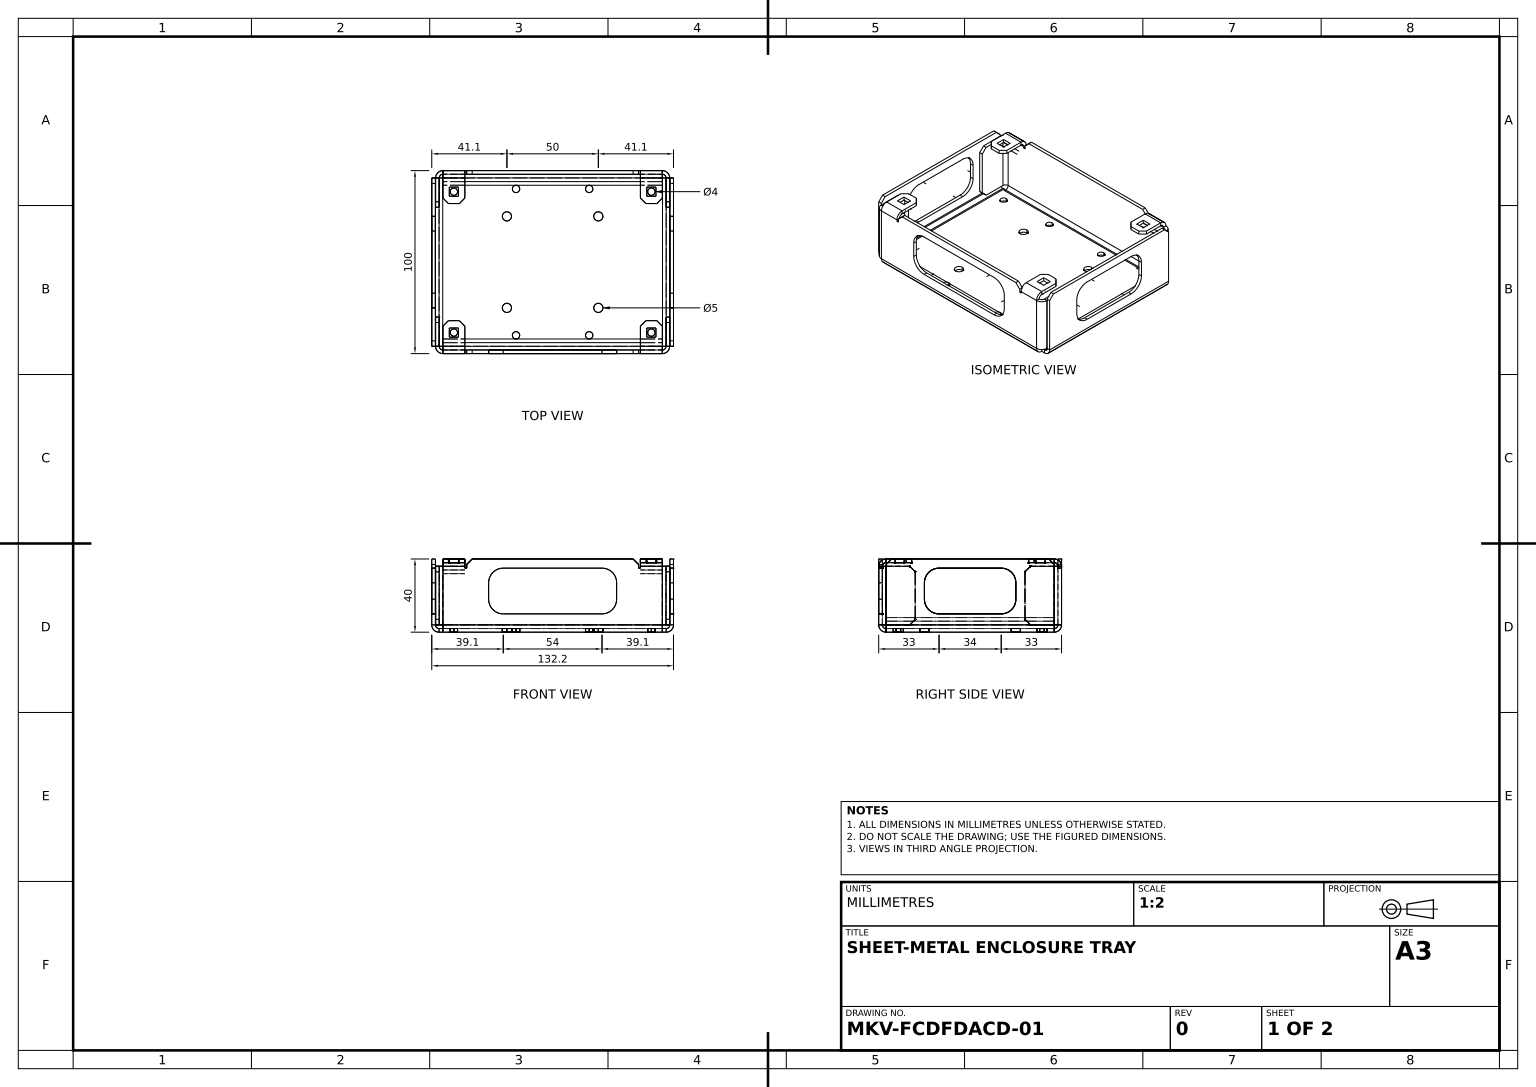
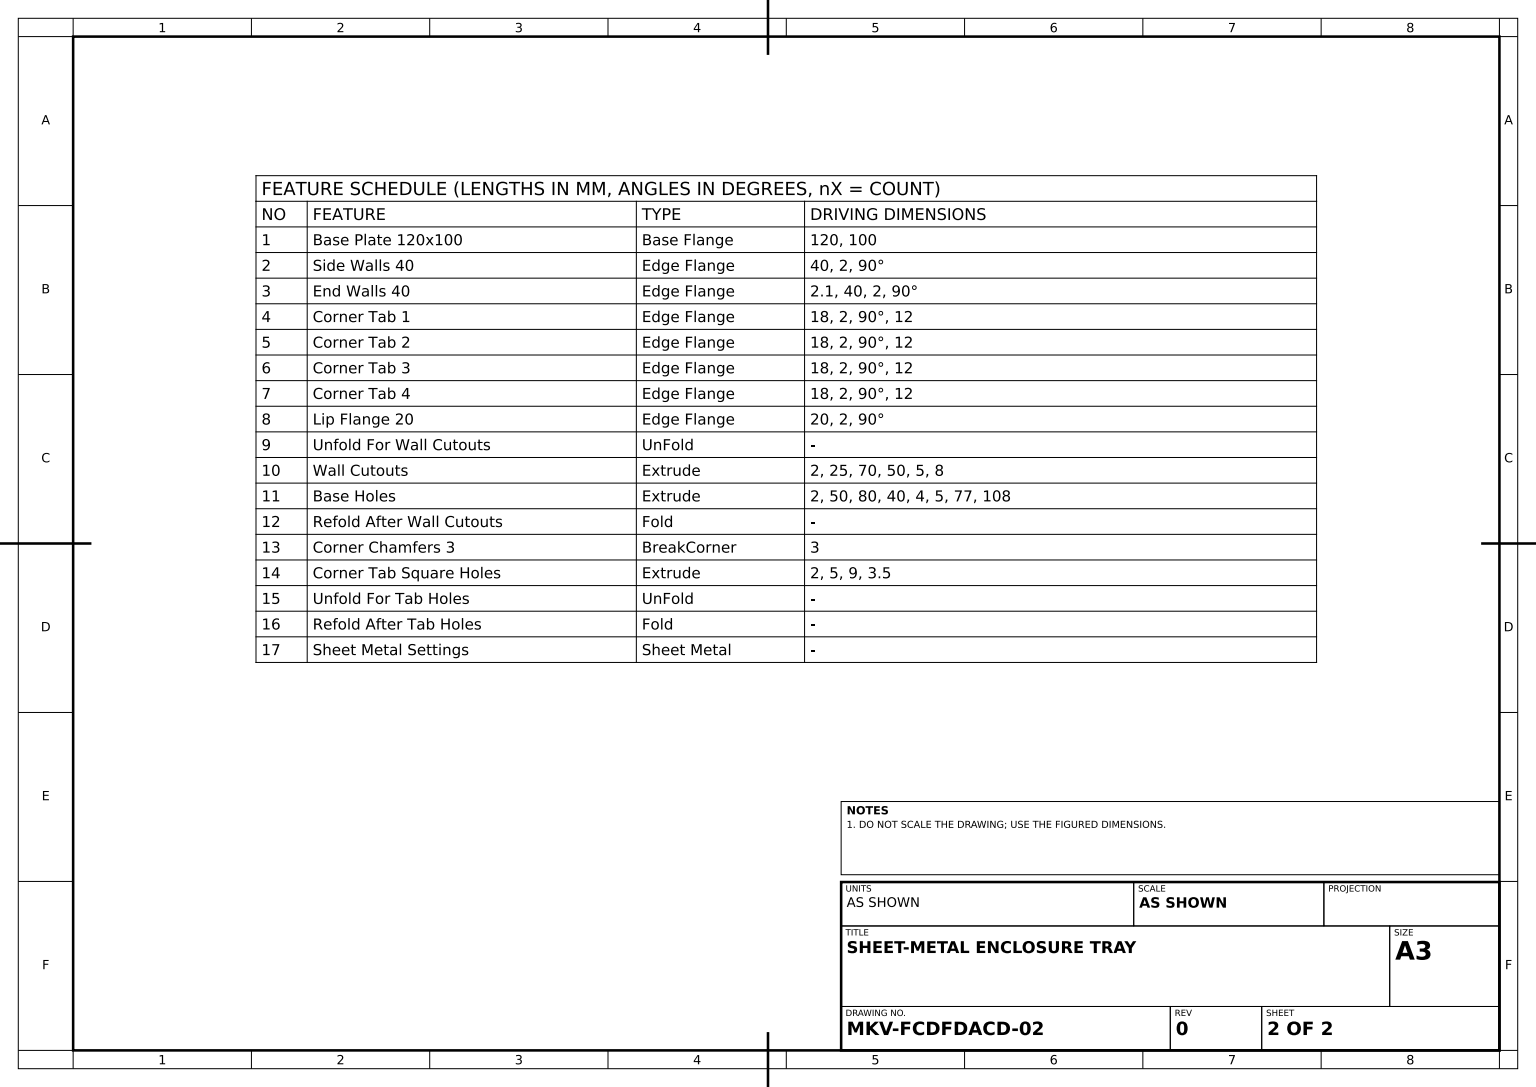
solid
v1 (-48,36,-48)
v2 (-48,38,-46)
e1 v1 v2 CIRCLE(AX(P(-48,36,-46),D(1,0,0),D(0,1,0)),2)
v3 (-48,36,-50)
e2 v1 v3 LINE
v4 (-48,40,-46)
e3 v3 v4 CIRCLE(AX(P(-48,36,-46),D(1,0,0),D(0,-1,0)),4)
e4 v2 v4 LINE
face PLANE(AX(P(-48,36,-46),D(-1,0,0),D(0,-1,0))) rev [-e1 e2 e3 -e4]
v5 (-48,38,46)
v6 (-48,36,48)
e5 v5 v6 CIRCLE(AX(P(-48,36,46),D(1,0,0),D(0,-1,0)),2)
v7 (-48,40,46)
e6 v5 v7 LINE
v8 (-48,36,50)
e7 v7 v8 CIRCLE(AX(P(-48,36,46),D(1,0,0),D(0,0,-1)),4)
e8 v6 v8 LINE
face PLANE(AX(P(-48,36,46),D(-1,0,0),D(0,1,0))) rev [-e5 e6 e7 -e8]
v9 (56.5,38,-41)
v10 (51.5,38,-41)
e9 v9 v10 LINE
v11 (56.5,40,-41)
e10 v9 v11 LINE
v12 (51.5,40,-41)
e11 v11 v12 LINE
e12 v10 v12 LINE
face PLANE(AX(P(56.5,38,-41),D(0,0,-1),D(0,1,0))) rev [-e9 e10 e11 -e12]
v13 (35,27,50)
v14 (35,27,48)
e13 v13 v14 LINE
v15 (35,18,48)
e14 v15 v14 LINE
v16 (35,18,50)
e15 v16 v15 LINE
e16 v16 v13 LINE
face PLANE(AX(P(35,-46.712389,50),D(-1,0,0),D(0,1,0))) [e13 -e14 -e15 e16]
v17 (-62,7,-30)
v18 (-62,4,-33)
e17 v17 v18 LINE
v19 (-64,7,-30)
e18 v19 v17 LINE
v20 (-64,4,-33)
e19 v20 v19 LINE
e20 v18 v20 LINE
face PLANE(AX(P(-64,7,-30),D(0,0.707106781,-0.707106781),D(1,0,0))) rev [-e17 -e18 -e19 -e20]
v21 (48,35,-48)
v22 (48,35,-50)
e21 v21 v22 LINE
v23 (47,35,-50)
e22 v22 v23 LINE
v24 (47,35,-48)
e23 v24 v23 LINE
e24 v24 v21 LINE
face PLANE(AX(P(47,35,-48),D(0,1,0),D(0,0,1))) [e21 e22 -e23 e24]
v25 (66.1,10,17)
v26 (64.1,10,17)
e25 v25 v26 LINE
v27 (64.1,18,25)
e26 v27 v26 CIRCLE(AX(P(64.1,18,17),D(1,0,0),D(0,0,1)),8)
v28 (66.1,18,25)
e27 v28 v27 LINE
e28 v28 v25 CIRCLE(AX(P(66.1,18,17),D(1,0,0),D(0,0,1)),8)
face CYL(AX(P(66.1,18,17),D(-1,0,0),D(0,0,1)),8) rev [e25 -e26 -e27 e28]
v29 (60,0,-46)
v30 (60,4,-50)
e29 v29 v30 CIRCLE(AX(P(60,4,-46),D(1,0,0),D(0,0,1)),4)
v31 (60,4,-48)
e30 v31 v30 LINE
v32 (60,2,-46)
e31 v32 v31 CIRCLE(AX(P(60,4,-46),D(1,0,0),D(0,0,-1)),2)
e32 v32 v29 LINE
face PLANE(AX(P(60,4,-46),D(-1,0,0),D(0,0,1))) rev [e29 -e30 -e31 e32]
v33 (54,0,-40.5)
v34 (54,0,-36.5)
e33 v33 v34 CIRCLE(AX(P(54,0,-38.5),D(0,1,0),D(0,0,1)),2)
v35 (54,2,-40.5)
e34 v33 v35 LINE
v36 (54,2,-36.5)
e35 v35 v36 CIRCLE(AX(P(54,2,-38.5),D(0,1,0),D(0,0,1)),2)
e36 v34 v36 LINE
face CYL(AX(P(54,0,-38.5),D(0,1,0),D(0,0,1)),2) rev [-e33 e34 e35 -e36]
v37 (57,38,-32)
v38 (57,40,-32)
e37 v37 v38 LINE
v39 (60,38,-35)
e38 v39 v37 LINE
v40 (60,40,-35)
e39 v40 v39 LINE
e40 v38 v40 LINE
face PLANE(AX(P(60,40,-35),D(-0.707106781,0,-0.707106781),D(0,-1,0))) rev [-e37 -e38 -e39 -e40]
v41 (51,40,32)
v42 (48,40,35)
e41 v41 v42 LINE
v43 (51,38,32)
e42 v43 v41 LINE
v44 (48,38,35)
e43 v44 v43 LINE
e44 v42 v44 LINE
face PLANE(AX(P(48,40,35),D(0.707106781,0,0.707106781),D(0,-1,0))) rev [-e41 -e42 -e43 -e44]
v45 (-51,38,32)
v46 (-57,38,32)
e45 v45 v46 LINE
v47 (-57,40,32)
e46 v46 v47 LINE
v48 (-51,40,32)
e47 v48 v47 LINE
e48 v48 v45 LINE
face PLANE(AX(P(-60,40,32),D(0,0,1),D(0,-1,0))) rev [e45 e46 -e47 e48]
v49 (64,36,-33)
v50 (64,33,-30)
e49 v49 v50 LINE
v51 (62,36,-33)
e50 v51 v49 LINE
v52 (62,33,-30)
e51 v52 v51 LINE
e52 v50 v52 LINE
face PLANE(AX(P(64,33,-30),D(0,-0.707106781,-0.707106781),D(-1,0,0))) rev [-e49 -e50 -e51 -e52]
v53 (-51,38,-32)
v54 (-51,40,-32)
e53 v53 v54 LINE
v55 (-57,40,-32)
e54 v55 v54 LINE
v56 (-57,38,-32)
e55 v55 v56 LINE
e56 v56 v53 LINE
face PLANE(AX(P(-48,40,-32),D(0,0,-1),D(0,1,0))) rev [e53 -e54 e55 e56]
v57 (-20,2,42)
v58 (-20,2,38)
e57 v57 v58 CIRCLE(AX(P(-20,2,40),D(0,1,0),D(0,0,1)),2)
v59 (-20,0,38)
e58 v59 v58 LINE
v60 (-20,0,42)
e59 v60 v59 CIRCLE(AX(P(-20,0,40),D(0,1,0),D(0,0,1)),2)
e60 v60 v57 LINE
face CYL(AX(P(-20,0,40),D(0,1,0),D(0,0,1)),2) rev [e57 -e58 -e59 e60]
v61 (-62,4,33)
v62 (-62,4,46)
e61 v61 v62 LINE
v63 (-62,7,30)
e62 v61 v63 LINE
v64 (-62,33,30)
e63 v64 v63 LINE
v65 (-62,36,33)
e64 v64 v65 LINE
v66 (-62,36,46)
e65 v66 v65 LINE
e66 v62 v66 LINE
face PLANE(AX(P(-62,0,0),D(1,0,0),D(0,0,-1))) [-e61 e62 -e63 e64 -e65 -e66]
v67 (-56.5,38,-36)
v68 (-56.5,40,-36)
e67 v67 v68 LINE
v69 (-51.5,40,-36)
e68 v68 v69 LINE
v70 (-51.5,38,-36)
e69 v70 v69 LINE
e70 v67 v70 LINE
face PLANE(AX(P(-56.5,38,-36),D(0,0,1),D(0,-1,0))) rev [e67 e68 -e69 -e70]
v71 (56.5,38,-36)
e71 v71 v9 LINE
v72 (51.5,38,-36)
e72 v10 v72 LINE
e73 v72 v71 LINE
v73 (48,38,-46)
v74 (48,38,-35)
e74 v73 v74 LINE
v75 (60,38,-46)
e75 v75 v73 LINE
e76 v39 v75 LINE
v76 (51,38,-32)
e77 v76 v37 LINE
e78 v76 v74 LINE
face PLANE(AX(P(0,38,0),D(0,-1,0),D(0,0,-1))) [e71 e9 e72 e73] [-e74 -e75 -e76 e38 -e77 e78]
v77 (48,40,46)
e79 v42 v77 LINE
v78 (48,38,46)
e80 v44 v78 LINE
e81 v78 v77 LINE
face PLANE(AX(P(48,40,48),D(1,0,0),D(0,0,-1))) rev [-e79 e44 e80 e81]
v79 (62,4,33)
v80 (64,4,33)
e82 v79 v80 LINE
v81 (64,4,46)
e83 v81 v80 LINE
v82 (62,4,46)
e84 v82 v81 LINE
e85 v82 v79 LINE
face PLANE(AX(P(64,4,30),D(0,1,0),D(0,0,1))) rev [e82 -e83 -e84 e85]
v83 (-60,4,48)
e86 v83 v62 CIRCLE(AX(P(-60,4,46),D(0,-1,0),D(0,0,-1)),2)
v84 (-60,4,50)
e87 v83 v84 LINE
v85 (-64,4,46)
e88 v84 v85 CIRCLE(AX(P(-60,4,46),D(0,-1,0),D(0,0,1)),4)
e89 v62 v85 LINE
face PLANE(AX(P(-60,4,46),D(0,1,0),D(0,0,1))) rev [-e86 e87 e88 -e89]
v86 (66.1,10,-17)
v87 (64.1,10,-17)
e90 v86 v87 LINE
e91 v87 v26 LINE
e92 v86 v25 LINE
face PLANE(AX(P(66.1,10,0),D(0,-1,0),D(0,0,1))) rev [e90 e91 -e25 -e92]
v88 (60,38,46)
e93 v78 v88 LINE
v89 (57,38,32)
e94 v89 v43 LINE
v90 (60,38,35)
e95 v89 v90 LINE
e96 v88 v90 LINE
v91 (51.5,38,41)
v92 (56.5,38,41)
e97 v91 v92 LINE
v93 (56.5,38,36)
e98 v92 v93 LINE
v94 (51.5,38,36)
e99 v93 v94 LINE
e100 v94 v91 LINE
face PLANE(AX(P(0,38,0),D(0,-1,0),D(0,0,-1))) [-e93 -e80 e43 -e94 e95 -e96] [e97 e98 e99 e100]
v95 (62,7,-30)
e101 v52 v95 LINE
v96 (64,7,-30)
e102 v95 v96 LINE
e103 v50 v96 LINE
face PLANE(AX(P(64,4,-30),D(0,0,-1),D(-1,0,0))) rev [e101 e102 -e103 e52]
v97 (56.5,40,36)
e104 v93 v97 LINE
v98 (56.5,40,41)
e105 v92 v98 LINE
e106 v98 v97 LINE
face PLANE(AX(P(56.5,38,41),D(1,0,0),D(0,0,-1))) rev [-e104 -e98 e105 e106]
v99 (-54,0,-40.5)
v100 (-54,0,-36.5)
e107 v99 v100 CIRCLE(AX(P(-54,0,-38.5),D(0,1,0),D(0,0,1)),2)
v101 (-54,2,-40.5)
e108 v99 v101 LINE
v102 (-54,2,-36.5)
e109 v101 v102 CIRCLE(AX(P(-54,2,-38.5),D(0,1,0),D(0,0,1)),2)
e110 v100 v102 LINE
face CYL(AX(P(-54,0,-38.5),D(0,1,0),D(0,0,1)),2) rev [-e107 e108 e109 -e110]
v103 (-54,0,36.5)
v104 (-54,2,36.5)
e111 v103 v104 LINE
v105 (-54,0,40.5)
e112 v105 v103 CIRCLE(AX(P(-54,0,38.5),D(0,1,0),D(0,0,1)),2)
v106 (-54,2,40.5)
e113 v105 v106 LINE
e114 v106 v104 CIRCLE(AX(P(-54,2,38.5),D(0,1,0),D(0,0,1)),2)
face CYL(AX(P(-54,0,38.5),D(0,1,0),D(0,0,1)),2) rev [-e111 -e112 e113 e114]
v107 (54,2,36.5)
v108 (54,2,40.5)
e115 v107 v108 CIRCLE(AX(P(54,2,38.5),D(0,1,0),D(0,0,1)),2)
e116 v108 v107 CIRCLE(AX(P(54,2,38.5),D(0,1,0),D(0,0,1)),2)
v109 (25,2,-27.5)
v110 (25,2,-22.5)
e117 v109 v110 CIRCLE(AX(P(25,2,-25),D(0,1,0),D(0,0,1)),2.5)
e118 v110 v109 CIRCLE(AX(P(25,2,-25),D(0,1,0),D(0,0,1)),2.5)
e119 v36 v35 CIRCLE(AX(P(54,2,-38.5),D(0,1,0),D(0,0,1)),2)
e120 v58 v57 CIRCLE(AX(P(-20,2,40),D(0,1,0),D(0,0,1)),2)
v111 (20,2,42)
v112 (20,2,38)
e121 v111 v112 CIRCLE(AX(P(20,2,40),D(0,1,0),D(0,0,1)),2)
e122 v112 v111 CIRCLE(AX(P(20,2,40),D(0,1,0),D(0,0,1)),2)
e123 v104 v106 CIRCLE(AX(P(-54,2,38.5),D(0,1,0),D(0,0,1)),2)
v113 (-25,2,22.5)
v114 (-25,2,27.5)
e124 v113 v114 CIRCLE(AX(P(-25,2,25),D(0,1,0),D(0,0,1)),2.5)
e125 v114 v113 CIRCLE(AX(P(-25,2,25),D(0,1,0),D(0,0,1)),2.5)
v115 (-25,2,-22.5)
v116 (-25,2,-27.5)
e126 v115 v116 CIRCLE(AX(P(-25,2,-25),D(0,1,0),D(0,0,1)),2.5)
e127 v116 v115 CIRCLE(AX(P(-25,2,-25),D(0,1,0),D(0,0,1)),2.5)
v117 (-20,2,-38)
v118 (-20,2,-42)
e128 v117 v118 CIRCLE(AX(P(-20,2,-40),D(0,1,0),D(0,0,1)),2)
e129 v118 v117 CIRCLE(AX(P(-20,2,-40),D(0,1,0),D(0,0,1)),2)
e130 v102 v101 CIRCLE(AX(P(-54,2,-38.5),D(0,1,0),D(0,0,1)),2)
v119 (62.1,2,-46)
v120 (62.1,2,46)
e131 v119 v120 LINE
e132 v119 v32 LINE
v121 (-60,2,-46)
e133 v121 v32 LINE
v122 (-62.1,2,-46)
e134 v122 v121 LINE
v123 (-62.1,2,46)
e135 v123 v122 LINE
v124 (-60,2,46)
e136 v123 v124 LINE
v125 (60,2,46)
e137 v125 v124 LINE
e138 v120 v125 LINE
v126 (20,2,-38)
v127 (20,2,-42)
e139 v126 v127 CIRCLE(AX(P(20,2,-40),D(0,1,0),D(0,0,1)),2)
e140 v127 v126 CIRCLE(AX(P(20,2,-40),D(0,1,0),D(0,0,1)),2)
v128 (25,2,22.5)
v129 (25,2,27.5)
e141 v128 v129 CIRCLE(AX(P(25,2,25),D(0,1,0),D(0,0,1)),2.5)
e142 v129 v128 CIRCLE(AX(P(25,2,25),D(0,1,0),D(0,0,1)),2.5)
face PLANE(AX(P(0,2,0),D(0,1,0),D(0,0,1))) [-e115 -e116] [-e117 -e118] [-e119 -e35] [-e120 -e57] [-e121 -e122] [-e123 -e114] [-e124 -e125] [-e126 -e127] [-e128 -e129] [-e109 -e130] [-e131 e132 -e133 -e134 -e135 e136 -e137 -e138] [-e139 -e140] [-e141 -e142]
v130 (-64.1,37,-46)
v131 (-64.1,40,-43)
e143 v130 v131 LINE
v132 (-66.1,37,-46)
e144 v132 v130 LINE
v133 (-66.1,40,-43)
e145 v133 v132 LINE
e146 v131 v133 LINE
face PLANE(AX(P(-66.1,37,-46),D(0,-0.707106781,0.707106781),D(1,0,0))) rev [-e143 -e144 -e145 -e146]
e147 v59 v60 CIRCLE(AX(P(-20,0,40),D(0,1,0),D(0,0,1)),2)
face CYL(AX(P(-20,0,40),D(0,1,0),D(0,0,1)),2) rev [-e147 e58 e120 -e60]
v134 (-60,40,46)
e148 v7 v134 LINE
v135 (-60,36,50)
e149 v135 v134 CIRCLE(AX(P(-60,36,46),D(-1,0,0),D(0,0,-1)),4)
e150 v8 v135 LINE
face CYL(AX(P(-67.046326,36,46),D(1,0,0),D(0,0,-1)),4) [e148 -e149 -e150 -e7]
v136 (-62,4,-46)
v137 (-64,4,-46)
e151 v136 v137 LINE
e152 v136 v18 LINE
e153 v137 v20 LINE
face PLANE(AX(P(-64,4,-30),D(0,1,0),D(0,0,1))) rev [-e151 e152 e20 -e153]
v138 (48,36,-48)
v139 (60,36,-48)
e154 v138 v139 LINE
e155 v139 v75 CIRCLE(AX(P(60,36,-46),D(1,0,0),D(0,1,0)),2)
e156 v73 v138 CIRCLE(AX(P(48,36,-46),D(-1,0,0),D(0,-1,0)),2)
face CYL(AX(P(67.046326,36,-46),D(-1,0,0),D(0,0,-1)),2) rev [e154 e155 e75 e156]
v140 (-60,4,-48)
e157 v31 v140 LINE
e158 v140 v121 CIRCLE(AX(P(-60,4,-46),D(-1,0,0),D(0,0,1)),2)
face CYL(AX(P(120.109145,4,-46),D(-1,0,0),D(0,0,1)),2) rev [e157 e158 e133 e31]
v141 (-48,35,-48)
e159 v1 v141 LINE
v142 (-48,35,-50)
e160 v141 v142 LINE
e161 v142 v3 LINE
face PLANE(AX(P(-48,36,-48),D(1,0,0),D(0,0,-1))) [-e2 e159 e160 e161]
v143 (60,40,-46)
e162 v75 v143 LINE
e163 v40 v143 LINE
face PLANE(AX(P(60,40,-48),D(-1,0,0),D(0,0,1))) rev [e162 -e163 e39 e76]
v144 (48,36,48)
v145 (48,35,48)
e164 v144 v145 LINE
v146 (48,35,50)
e165 v145 v146 LINE
v147 (48,36,50)
e166 v146 v147 LINE
e167 v144 v147 LINE
face PLANE(AX(P(48,36,48),D(-1,0,0),D(0,0,1))) [e164 e165 e166 -e167]
v148 (64.1,4,46)
e168 v120 v148 CIRCLE(AX(P(62.1,4,46),D(0,0,1),D(1,0,0)),2)
v149 (62.1,0,46)
e169 v120 v149 LINE
v150 (66.1,4,46)
e170 v149 v150 CIRCLE(AX(P(62.1,4,46),D(0,0,1),D(-1,0,0)),4)
e171 v148 v150 LINE
face PLANE(AX(P(62.1,4,46),D(0,0,-1),D(-1,0,0))) rev [-e168 e169 e170 -e171]
v151 (-66.1,37,46)
v152 (-66.1,40,43)
e172 v151 v152 LINE
e173 v152 v133 LINE
v153 (-66.1,4,-46)
e174 v132 v153 LINE
v154 (-66.1,4,46)
e175 v154 v153 LINE
e176 v154 v151 LINE
v155 (-66.1,35,-17)
v156 (-66.1,35,17)
e177 v155 v156 LINE
v157 (-66.1,27,25)
e178 v156 v157 CIRCLE(AX(P(-66.1,27,17),D(1,0,0),D(0,0,1)),8)
v158 (-66.1,18,25)
e179 v157 v158 LINE
v159 (-66.1,10,17)
e180 v158 v159 CIRCLE(AX(P(-66.1,18,17),D(1,0,0),D(0,0,1)),8)
v160 (-66.1,10,-17)
e181 v160 v159 LINE
v161 (-66.1,18,-25)
e182 v161 v160 CIRCLE(AX(P(-66.1,18,-17),D(-1,0,0),D(0,0,1)),8)
v162 (-66.1,27,-25)
e183 v162 v161 LINE
e184 v162 v155 CIRCLE(AX(P(-66.1,27,-17),D(1,0,0),D(0,0,1)),8)
face PLANE(AX(P(-66.1,0,0),D(1,0,0),D(0,1,0))) rev [e172 e173 e145 e174 -e175 e176] [e177 e178 e179 e180 -e181 -e182 -e183 e184]
v163 (51.5,40,41)
e185 v91 v163 LINE
e186 v163 v98 LINE
face PLANE(AX(P(56.5,38,41),D(0,0,1),D(0,-1,0))) rev [-e97 e185 e186 -e105]
v164 (-47,37,48)
v165 (-47,35,48)
e187 v164 v165 LINE
v166 (-47,35,50)
e188 v165 v166 LINE
v167 (-47,37,50)
e189 v166 v167 LINE
e190 v167 v164 LINE
face PLANE(AX(P(-47,40,48),D(-1,0,0),D(0,0,1))) [e187 e188 e189 e190]
v168 (60,4,50)
e191 v81 v168 CIRCLE(AX(P(60,4,46),D(0,-1,0),D(0,0,-1)),4)
v169 (60,4,48)
e192 v169 v168 LINE
e193 v82 v169 CIRCLE(AX(P(60,4,46),D(0,-1,0),D(-1,0,0)),2)
face PLANE(AX(P(60,4,46),D(0,1,0),D(1,0,0))) rev [e84 e191 -e192 -e193]
v170 (-25,0,27.5)
v171 (-25,0,22.5)
e194 v170 v171 CIRCLE(AX(P(-25,0,25),D(0,1,0),D(0,0,1)),2.5)
e195 v170 v114 LINE
e196 v171 v113 LINE
face CYL(AX(P(-25,0,25),D(0,1,0),D(0,0,1)),2.5) rev [-e194 e195 e125 -e196]
v172 (-62.1,0,-46)
e197 v172 v153 CIRCLE(AX(P(-62.1,4,-46),D(0,0,-1),D(1,0,0)),4)
v173 (-62.1,0,46)
e198 v173 v172 LINE
e199 v154 v173 CIRCLE(AX(P(-62.1,4,46),D(0,0,1),D(1,0,0)),4)
face CYL(AX(P(-62.1,4,-92.142317),D(0,0,1),D(1,0,0)),4) [e175 -e197 -e198 -e199]
v174 (66.1,35,-17)
v175 (66.1,35,17)
e200 v174 v175 LINE
v176 (64.1,35,17)
e201 v175 v176 LINE
v177 (64.1,35,-17)
e202 v177 v176 LINE
e203 v174 v177 LINE
face PLANE(AX(P(66.1,35,0),D(0,-1,0),D(0,0,1))) [e200 e201 -e202 -e203]
v178 (-60,4,-50)
e204 v140 v178 LINE
v179 (-60,0,-46)
e205 v178 v179 CIRCLE(AX(P(-60,4,-46),D(-1,0,0),D(0,0,1)),4)
e206 v121 v179 LINE
face PLANE(AX(P(-60,4,-46),D(1,0,0),D(0,0,-1))) rev [e204 e205 -e206 -e158]
v180 (-60,38,35)
e207 v180 v46 LINE
v181 (-60,40,35)
e208 v181 v180 LINE
e209 v47 v181 LINE
face PLANE(AX(P(-60,40,35),D(0.707106781,0,0.707106781),D(0,-1,0))) rev [-e46 -e207 -e208 -e209]
v182 (-64,36,-33)
v183 (-64,36,-46)
e210 v182 v183 LINE
e211 v137 v183 LINE
v184 (-64,33,-30)
e212 v19 v184 LINE
e213 v184 v182 LINE
face PLANE(AX(P(-64,0,0),D(1,0,0),D(0,0,-1))) rev [e210 -e211 e153 e19 e212 e213]
v185 (62,4,-46)
v186 (64,4,-46)
e214 v185 v186 LINE
e215 v31 v185 CIRCLE(AX(P(60,4,-46),D(0,-1,0),D(0,0,-1)),2)
e216 v30 v186 CIRCLE(AX(P(60,4,-46),D(0,-1,0),D(0,0,1)),4)
face PLANE(AX(P(60,4,-46),D(0,1,0),D(0,0,1))) rev [-e214 -e215 e30 e216]
v187 (60,36,48)
e217 v187 v144 LINE
e218 v144 v78 CIRCLE(AX(P(48,36,46),D(-1,0,0),D(0,1,0)),2)
e219 v88 v187 CIRCLE(AX(P(60,36,46),D(1,0,0),D(0,-1,0)),2)
face CYL(AX(P(40.953674,36,46),D(1,0,0),D(0,-1,0)),2) rev [e217 e218 e93 e219]
v188 (-47,37,-50)
v189 (-47,35,-50)
e220 v188 v189 LINE
v190 (-47,35,-48)
e221 v190 v189 LINE
v191 (-47,37,-48)
e222 v190 v191 LINE
e223 v191 v188 LINE
face PLANE(AX(P(-47,35,-48),D(-1,0,0),D(0,0,1))) [e220 -e221 e222 e223]
v192 (60,36,-50)
e224 v139 v192 LINE
e225 v192 v143 CIRCLE(AX(P(60,36,-46),D(1,0,0),D(0,0,-1)),4)
face PLANE(AX(P(60,36,-46),D(-1,0,0),D(0,-1,0))) rev [-e155 e224 e225 -e162]
v193 (60,0,46)
e226 v149 v193 LINE
e227 v125 v193 LINE
face PLANE(AX(P(62.1,2,46),D(0,0,-1),D(0,-1,0))) rev [-e226 -e169 e138 e227]
v194 (-44,40,-48)
e228 v194 v191 LINE
v195 (-44,40,-50)
e229 v195 v194 LINE
e230 v188 v195 LINE
face PLANE(AX(P(-47,37,-48),D(-0.707106781,0.707106781,0),D(0,0,1))) [-e223 -e228 -e229 -e230]
v196 (-62,36,-46)
e231 v196 v183 LINE
v197 (-60,36,-48)
e232 v197 v196 CIRCLE(AX(P(-60,36,-46),D(0,1,0),D(0,0,1)),2)
v198 (-60,36,-50)
e233 v197 v198 LINE
e234 v198 v183 CIRCLE(AX(P(-60,36,-46),D(0,1,0),D(0,0,-1)),4)
face PLANE(AX(P(-60,36,-46),D(0,-1,0),D(0,0,-1))) rev [-e231 -e232 e233 e234]
e235 v124 v83 CIRCLE(AX(P(-60,4,46),D(-1,0,0),D(0,0,1)),2)
v199 (-60,0,46)
e236 v124 v199 LINE
e237 v199 v84 CIRCLE(AX(P(-60,4,46),D(-1,0,0),D(0,0,-1)),4)
face PLANE(AX(P(-60,4,46),D(1,0,0),D(0,0,-1))) rev [-e235 e236 e237 -e87]
v200 (57,40,32)
e238 v200 v89 LINE
e239 v200 v41 LINE
face PLANE(AX(P(48,40,32),D(0,0,1),D(0,-1,0))) rev [e238 e94 e42 -e239]
v201 (-25,0,-22.5)
e240 v201 v115 LINE
v202 (-25,0,-27.5)
e241 v202 v201 CIRCLE(AX(P(-25,0,-25),D(0,1,0),D(0,0,1)),2.5)
e242 v202 v116 LINE
face CYL(AX(P(-25,0,-25),D(0,1,0),D(0,0,1)),2.5) rev [-e240 -e241 e242 e127]
v203 (-64.1,4,46)
e243 v203 v123 CIRCLE(AX(P(-62.1,4,46),D(0,0,1),D(1,0,0)),2)
v204 (-64.1,4,-46)
e244 v122 v204 CIRCLE(AX(P(-62.1,4,-46),D(0,0,-1),D(-1,0,0)),2)
e245 v204 v203 LINE
face CYL(AX(P(-62.1,4,-92.142317),D(0,0,1),D(1,0,0)),2) rev [e243 e135 e244 e245]
v205 (62.1,0,-46)
e246 v119 v205 LINE
e247 v205 v29 LINE
face PLANE(AX(P(62.1,2,-46),D(0,0,-1),D(0,-1,0))) [e246 e247 -e32 -e132]
v206 (64,36,46)
e248 v81 v206 LINE
v207 (60,36,50)
e249 v207 v206 CIRCLE(AX(P(60,36,46),D(0,1,0),D(0,0,-1)),4)
e250 v168 v207 LINE
face CYL(AX(P(60,52.406891,46),D(0,-1,0),D(0,0,-1)),4) [e248 -e249 -e250 -e191]
v208 (66.1,37,46)
v209 (64.1,37,46)
e251 v208 v209 LINE
v210 (66.1,40,43)
e252 v210 v208 LINE
v211 (64.1,40,43)
e253 v211 v210 LINE
e254 v209 v211 LINE
face PLANE(AX(P(66.1,37,46),D(0,-0.707106781,-0.707106781),D(-1,0,0))) rev [-e251 -e252 -e253 -e254]
v212 (64.1,4,-46)
v213 (64.1,37,-46)
e255 v212 v213 LINE
v214 (66.1,37,-46)
e256 v213 v214 LINE
v215 (66.1,4,-46)
e257 v215 v214 LINE
e258 v212 v215 LINE
face PLANE(AX(P(66.1,40,-46),D(0,0,1),D(1,0,0))) rev [e255 e256 -e257 -e258]
v216 (-51.5,38,-41)
v217 (-56.5,38,-41)
e259 v216 v217 LINE
e260 v217 v67 LINE
e261 v70 v216 LINE
v218 (-60,38,-46)
e262 v2 v218 LINE
v219 (-48,38,-35)
e263 v219 v2 LINE
e264 v219 v53 LINE
v220 (-60,38,-35)
e265 v56 v220 LINE
e266 v218 v220 LINE
face PLANE(AX(P(0,38,0),D(0,-1,0),D(0,0,-1))) [e259 e260 e70 e261] [-e262 -e263 e264 -e56 e265 -e266]
e267 v196 v136 LINE
e268 v136 v140 CIRCLE(AX(P(-60,4,-46),D(0,-1,0),D(1,0,0)),2)
e269 v140 v197 LINE
face CYL(AX(P(-60,52.406891,-46),D(0,-1,0),D(0,0,-1)),2) rev [e232 e267 e268 e269]
v221 (51.5,40,36)
e270 v94 v221 LINE
e271 v221 v163 LINE
face PLANE(AX(P(51.5,38,41),D(-1,0,0),D(0,0,1))) rev [-e100 e270 e271 -e185]
v222 (-64.1,18,-25)
e272 v161 v222 LINE
v223 (-64.1,10,-17)
e273 v160 v223 LINE
e274 v222 v223 CIRCLE(AX(P(-64.1,18,-17),D(-1,0,0),D(0,0,1)),8)
face CYL(AX(P(-66.1,18,-17),D(1,0,0),D(0,0,1)),8) rev [-e272 e182 e273 -e274]
v224 (-51.5,38,41)
v225 (-51.5,38,36)
e275 v224 v225 LINE
v226 (-51.5,40,41)
e276 v224 v226 LINE
v227 (-51.5,40,36)
e277 v226 v227 LINE
e278 v225 v227 LINE
face PLANE(AX(P(-51.5,38,41),D(1,0,0),D(0,0,-1))) rev [-e275 e276 e277 -e278]
v228 (44,40,48)
v229 (-44,40,48)
e279 v228 v229 LINE
v230 (-44,40,50)
e280 v229 v230 LINE
v231 (44,40,50)
e281 v231 v230 LINE
e282 v231 v228 LINE
face PLANE(AX(P(-60,40,50),D(0,-1,0),D(0,0,-1))) rev [e279 e280 -e281 e282]
v232 (64,36,-46)
e283 v232 v192 CIRCLE(AX(P(60,36,-46),D(0,1,0),D(0,0,1)),4)
v233 (62,36,-46)
e284 v233 v139 CIRCLE(AX(P(60,36,-46),D(0,1,0),D(-1,0,0)),2)
e285 v233 v232 LINE
face PLANE(AX(P(60,36,-46),D(0,-1,0),D(1,0,0))) rev [e283 -e224 -e284 e285]
v234 (62,4,-33)
e286 v234 v95 LINE
e287 v233 v51 LINE
e288 v185 v233 LINE
e289 v234 v185 LINE
face PLANE(AX(P(62,0,0),D(-1,0,0),D(0,0,1))) [e286 -e101 e51 -e287 -e288 -e289]
v235 (25,0,27.5)
e290 v235 v129 LINE
v236 (25,0,22.5)
e291 v236 v235 CIRCLE(AX(P(25,0,25),D(0,1,0),D(0,0,1)),2.5)
e292 v236 v128 LINE
face CYL(AX(P(25,0,25),D(0,1,0),D(0,0,1)),2.5) rev [e141 -e290 -e291 e292]
e293 v100 v99 CIRCLE(AX(P(-54,0,-38.5),D(0,1,0),D(0,0,1)),2)
face CYL(AX(P(-54,0,-38.5),D(0,1,0),D(0,0,1)),2) rev [-e108 -e293 e110 e130]
v237 (51,40,-32)
e294 v237 v76 LINE
v238 (48,40,-35)
e295 v238 v237 LINE
e296 v74 v238 LINE
face PLANE(AX(P(51,40,-32),D(0.707106781,0,-0.707106781),D(0,-1,0))) rev [-e294 -e295 -e296 -e78]
v239 (64.1,27,25)
e297 v239 v27 LINE
v240 (66.1,27,25)
e298 v240 v239 LINE
e299 v240 v28 LINE
face PLANE(AX(P(66.1,-62.812389,25),D(0,0,-1),D(0,-1,0))) [e27 -e297 -e298 e299]
v241 (-64.1,27,25)
v242 (-64.1,18,25)
e300 v241 v242 LINE
e301 v158 v242 LINE
e302 v157 v241 LINE
face PLANE(AX(P(-66.1,-62.812389,25),D(0,0,1),D(0,-1,0))) rev [e300 -e301 -e179 e302]
e303 v237 v38 LINE
face PLANE(AX(P(60,40,-32),D(0,0,-1),D(0,1,0))) rev [e294 e77 e37 -e303]
v243 (-64.1,27,-25)
e304 v243 v222 LINE
e305 v162 v243 LINE
face PLANE(AX(P(-66.1,-62.812389,-25),D(0,0,1),D(0,-1,0))) [-e304 -e305 e183 e272]
e306 v207 v147 LINE
v244 (60,40,46)
e307 v244 v207 CIRCLE(AX(P(60,36,46),D(1,0,0),D(0,-1,0)),4)
e308 v244 v77 LINE
e309 v147 v77 CIRCLE(AX(P(48,36,46),D(-1,0,0),D(0,-1,0)),4)
face CYL(AX(P(40.953674,36,46),D(1,0,0),D(0,-1,0)),4) [-e306 -e307 e308 -e309]
v245 (60,40,35)
e310 v245 v200 LINE
e311 v90 v245 LINE
face PLANE(AX(P(57,40,32),D(-0.707106781,0,0.707106781),D(0,-1,0))) rev [-e95 -e238 -e310 -e311]
v246 (51.5,40,-36)
e312 v72 v246 LINE
v247 (56.5,40,-36)
e313 v246 v247 LINE
e314 v71 v247 LINE
face PLANE(AX(P(56.5,38,-36),D(0,0,1),D(0,-1,0))) rev [-e73 e312 e313 -e314]
v248 (-64,7,30)
v249 (-64,4,33)
e315 v248 v249 LINE
e316 v63 v248 LINE
e317 v249 v61 LINE
face PLANE(AX(P(-64,4,33),D(0,0.707106781,0.707106781),D(1,0,0))) rev [-e315 -e316 -e62 -e317]
e318 v189 v142 LINE
v250 (44,40,-50)
e319 v195 v250 LINE
v251 (47,37,-50)
e320 v250 v251 LINE
e321 v23 v251 LINE
v252 (48,36,-50)
e322 v252 v22 LINE
e323 v252 v192 LINE
e324 v192 v30 LINE
e325 v178 v30 LINE
e326 v178 v198 LINE
e327 v198 v3 LINE
face PLANE(AX(P(0,0,-50),D(0,0,1),D(0,-1,0))) rev [-e161 -e318 -e220 e230 e319 e320 -e321 -e22 -e322 e323 e324 -e325 e326 e327]
e328 v171 v170 CIRCLE(AX(P(-25,0,25),D(0,1,0),D(0,0,1)),2.5)
face CYL(AX(P(-25,0,25),D(0,1,0),D(0,0,1)),2.5) rev [-e328 e196 e124 -e195]
e329 v201 v202 CIRCLE(AX(P(-25,0,-25),D(0,1,0),D(0,0,1)),2.5)
face CYL(AX(P(-25,0,-25),D(0,1,0),D(0,0,1)),2.5) rev [e240 e126 -e242 -e329]
v253 (-64,33,30)
e330 v253 v64 LINE
v254 (-64,36,33)
e331 v254 v253 LINE
e332 v65 v254 LINE
face PLANE(AX(P(-64,33,30),D(0,-0.707106781,0.707106781),D(1,0,0))) rev [-e64 -e330 -e331 -e332]
e333 v141 v190 LINE
face PLANE(AX(P(-48,35,-48),D(0,1,0),D(0,0,1))) [e318 -e160 e333 e221]
v255 (66.1,40,-43)
v256 (64.1,40,-43)
e334 v255 v256 LINE
e335 v256 v211 LINE
e336 v255 v210 LINE
face PLANE(AX(P(66.1,40,46),D(0,-1,0),D(1,0,0))) rev [e334 e335 e253 -e336]
v257 (-27,10,50)
v258 (-35,18,50)
e337 v257 v258 CIRCLE(AX(P(-27,18,50),D(0,0,-1),D(0,1,0)),8)
v259 (-27,10,48)
e338 v257 v259 LINE
v260 (-35,18,48)
e339 v259 v260 CIRCLE(AX(P(-27,18,48),D(0,0,-1),D(0,1,0)),8)
e340 v258 v260 LINE
face CYL(AX(P(-27,18,50),D(0,0,-1),D(0,1,0)),8) rev [-e337 e338 e339 -e340]
v261 (47,37,48)
v262 (47,37,50)
e341 v261 v262 LINE
v263 (47,35,50)
e342 v262 v263 LINE
v264 (47,35,48)
e343 v264 v263 LINE
e344 v264 v261 LINE
face PLANE(AX(P(47,35,48),D(1,0,0),D(0,0,-1))) [e341 e342 -e343 e344]
e345 v175 v240 CIRCLE(AX(P(66.1,27,17),D(1,0,0),D(0,0,1)),8)
e346 v176 v239 CIRCLE(AX(P(64.1,27,17),D(1,0,0),D(0,0,1)),8)
face CYL(AX(P(66.1,27,17),D(-1,0,0),D(0,0,1)),8) rev [-e201 e345 e298 -e346]
v265 (64,7,30)
e347 v80 v265 LINE
v266 (64,33,30)
e348 v265 v266 LINE
v267 (64,36,33)
e349 v266 v267 LINE
e350 v267 v206 LINE
face PLANE(AX(P(64,0,0),D(-1,0,0),D(0,0,1))) rev [-e248 e83 e347 e348 e349 e350]
v268 (-64.1,35,17)
e351 v156 v268 LINE
e352 v268 v241 CIRCLE(AX(P(-64.1,27,17),D(1,0,0),D(0,0,1)),8)
face CYL(AX(P(-66.1,27,17),D(1,0,0),D(0,0,1)),8) rev [e351 e352 -e302 -e178]
e353 v244 v245 LINE
e354 v97 v221 LINE
face PLANE(AX(P(0,40,0),D(0,-1,0),D(0,0,-1))) rev [e239 e41 e79 -e308 e353 e310] [-e186 -e271 -e354 -e106]
v269 (64,4,-33)
e355 v96 v269 LINE
e356 v269 v186 LINE
e357 v232 v186 LINE
e358 v232 v49 LINE
face PLANE(AX(P(64,0,0),D(-1,0,0),D(0,0,1))) rev [e355 e356 -e357 e358 e49 e103]
e359 v122 v172 LINE
e360 v172 v179 LINE
face PLANE(AX(P(-62.1,2,-46),D(0,0,1),D(0,-1,0))) rev [-e359 e134 e206 -e360]
v270 (25,0,-27.5)
e361 v270 v109 LINE
v271 (25,0,-22.5)
e362 v271 v270 CIRCLE(AX(P(25,0,-25),D(0,1,0),D(0,0,1)),2.5)
e363 v271 v110 LINE
face CYL(AX(P(25,0,-25),D(0,1,0),D(0,0,1)),2.5) rev [-e361 -e362 e363 e118]
e364 v103 v105 CIRCLE(AX(P(-54,0,38.5),D(0,1,0),D(0,0,1)),2)
face CYL(AX(P(-54,0,38.5),D(0,1,0),D(0,0,1)),2) rev [e111 e123 -e113 -e364]
v272 (27,35,50)
v273 (27,35,48)
e365 v272 v273 LINE
v274 (-27,35,50)
e366 v274 v272 LINE
v275 (-27,35,48)
e367 v274 v275 LINE
e368 v275 v273 LINE
face PLANE(AX(P(0,35,50),D(0,1,0),D(1,0,0))) rev [-e365 -e366 e367 e368]
e369 v137 v178 CIRCLE(AX(P(-60,4,-46),D(0,-1,0),D(0,0,-1)),4)
face PLANE(AX(P(-60,4,-46),D(0,1,0),D(-1,0,0))) rev [-e204 -e268 e151 e369]
v276 (-48,35,50)
e370 v8 v276 LINE
v277 (-48,35,48)
e371 v277 v276 LINE
e372 v277 v6 LINE
face PLANE(AX(P(-48,35,48),D(1,0,0),D(0,0,-1))) [e8 e370 -e371 e372]
v278 (48,40,-46)
e373 v278 v238 LINE
e374 v73 v278 LINE
face PLANE(AX(P(48,40,-32),D(1,0,0),D(0,0,-1))) rev [e296 -e373 -e374 e74]
v279 (27,10,48)
e375 v259 v279 LINE
v280 (27,10,50)
e376 v257 v280 LINE
e377 v280 v279 LINE
face PLANE(AX(P(0,10,50),D(0,1,0),D(1,0,0))) [-e375 -e338 e376 e377]
v281 (-60,36,48)
e378 v66 v281 CIRCLE(AX(P(-60,36,46),D(0,1,0),D(0,0,1)),2)
v282 (-64,36,46)
e379 v66 v282 LINE
e380 v282 v135 CIRCLE(AX(P(-60,36,46),D(0,1,0),D(0,0,1)),4)
e381 v281 v135 LINE
face PLANE(AX(P(-60,36,46),D(0,-1,0),D(0,0,-1))) rev [-e378 e379 e380 -e381]
e382 v278 v252 CIRCLE(AX(P(48,36,-46),D(-1,0,0),D(0,0,-1)),4)
e383 v278 v143 LINE
face CYL(AX(P(67.046326,36,-46),D(-1,0,0),D(0,0,-1)),4) [-e382 e383 -e225 -e323]
e384 v269 v234 LINE
face PLANE(AX(P(64,4,-33),D(0,0.707106781,-0.707106781),D(-1,0,0))) rev [-e102 -e286 -e384 -e355]
v283 (62,7,30)
e385 v283 v79 LINE
e386 v265 v283 LINE
face PLANE(AX(P(64,7,30),D(0,0.707106781,0.707106781),D(-1,0,0))) rev [-e82 -e385 -e386 -e347]
v284 (62,36,46)
e387 v284 v206 LINE
e388 v187 v284 CIRCLE(AX(P(60,36,46),D(0,1,0),D(1,0,0)),2)
e389 v187 v207 LINE
face PLANE(AX(P(60,36,46),D(0,-1,0),D(-1,0,0))) rev [-e387 -e388 e389 e249]
e390 v214 v255 LINE
e391 v256 v213 LINE
face PLANE(AX(P(66.1,40,-43),D(0,-0.707106781,0.707106781),D(-1,0,0))) rev [-e390 -e256 -e391 -e334]
v285 (62,36,33)
e392 v267 v285 LINE
e393 v285 v284 LINE
face PLANE(AX(P(64,36,48),D(0,-1,0),D(0,0,-1))) rev [-e350 e392 e393 e387]
face PLANE(AX(P(64,36,-30),D(0,-1,0),D(0,0,-1))) rev [e50 -e358 -e285 e287]
v286 (-60,40,-35)
e394 v220 v286 LINE
v287 (-60,40,-46)
e395 v287 v286 LINE
e396 v218 v287 LINE
face PLANE(AX(P(-60,40,-32),D(1,0,0),D(0,0,-1))) rev [e266 e394 -e395 -e396]
v288 (44,40,-48)
e397 v194 v288 LINE
e398 v197 v1 LINE
e399 v139 v31 LINE
e400 v21 v138 LINE
v289 (47,37,-48)
e401 v289 v24 LINE
e402 v289 v288 LINE
face PLANE(AX(P(0,0,-48),D(0,0,1),D(0,-1,0))) [-e397 e228 -e222 -e333 -e159 -e398 -e269 -e157 -e399 -e154 -e400 -e24 -e401 e402]
e403 v262 v231 LINE
e404 v228 v261 LINE
face PLANE(AX(P(47,37,48),D(0.707106781,0.707106781,0),D(0,0,-1))) [-e282 -e403 -e341 -e404]
e405 v135 v84 LINE
e406 v282 v85 LINE
face CYL(AX(P(-60,-12.406891,46),D(0,1,0),D(0,0,1)),4) [-e405 -e380 e406 -e88]
v290 (-56.5,40,36)
e407 v227 v290 LINE
v291 (-56.5,38,36)
e408 v291 v290 LINE
e409 v225 v291 LINE
face PLANE(AX(P(-56.5,38,36),D(0,0,-1),D(0,1,0))) rev [e278 e407 -e408 -e409]
v292 (-51.5,40,-41)
v293 (-56.5,40,-41)
e410 v292 v293 LINE
e411 v69 v292 LINE
e412 v293 v68 LINE
e413 v287 v4 LINE
e414 v286 v55 LINE
v294 (-48,40,-35)
e415 v54 v294 LINE
e416 v294 v4 LINE
face PLANE(AX(P(0,40,0),D(0,-1,0),D(0,0,-1))) rev [-e410 -e411 -e68 -e412] [-e413 e395 e414 e54 e415 e416]
v295 (-56.5,38,41)
e417 v291 v295 LINE
v296 (-56.5,40,41)
e418 v290 v296 LINE
e419 v295 v296 LINE
face PLANE(AX(P(-56.5,38,41),D(-1,0,0),D(0,0,1))) rev [-e417 e408 e418 -e419]
e420 v247 v11 LINE
e421 v12 v246 LINE
face PLANE(AX(P(0,40,0),D(0,-1,0),D(0,0,-1))) rev [-e420 -e313 -e421 -e11] [e303 e40 e163 -e383 e373 e295]
e422 v282 v254 LINE
face PLANE(AX(P(-64,36,30),D(0,-1,0),D(0,0,-1))) rev [-e379 e65 e332 -e422]
e423 v164 v229 LINE
e424 v230 v167 LINE
face PLANE(AX(P(-44,40,50),D(-0.707106781,0.707106781,0),D(0,0,-1))) [-e423 -e190 -e424 -e280]
v297 (64.1,27,-25)
v298 (64.1,18,-25)
e425 v297 v298 LINE
v299 (66.1,18,-25)
e426 v299 v298 LINE
v300 (66.1,27,-25)
e427 v300 v299 LINE
e428 v300 v297 LINE
face PLANE(AX(P(66.1,-62.812389,-25),D(0,0,-1),D(0,-1,0))) rev [e425 -e426 -e427 e428]
e429 v145 v264 LINE
e430 v169 v187 LINE
e431 v83 v169 LINE
e432 v281 v83 LINE
e433 v6 v281 LINE
e434 v165 v277 LINE
e435 v279 v15 CIRCLE(AX(P(27,18,48),D(0,0,1),D(0,1,0)),8)
e436 v273 v14 CIRCLE(AX(P(27,27,48),D(0,0,-1),D(0,1,0)),8)
v301 (-35,27,48)
e437 v301 v275 CIRCLE(AX(P(-27,27,48),D(0,0,-1),D(0,1,0)),8)
e438 v260 v301 LINE
face PLANE(AX(P(0,0,48),D(0,0,-1),D(-1,0,0))) [-e187 e423 -e279 e404 -e344 -e429 -e164 -e217 -e430 -e431 -e432 -e433 -e372 -e434] [e375 e435 e14 -e436 -e368 -e437 -e438 -e339]
e439 v276 v166 LINE
face PLANE(AX(P(-47,35,48),D(0,1,0),D(0,0,1))) [e371 e439 -e188 e434]
v302 (-62,33,-30)
e440 v17 v302 LINE
e441 v302 v184 LINE
face PLANE(AX(P(-64,36,-30),D(0,0,-1),D(-1,0,0))) rev [e18 e440 e441 -e212]
v303 (20,0,-38)
e442 v303 v126 LINE
v304 (20,0,-42)
e443 v304 v127 LINE
e444 v303 v304 CIRCLE(AX(P(20,0,-40),D(0,1,0),D(0,0,1)),2)
face CYL(AX(P(20,0,-40),D(0,1,0),D(0,0,1)),2) rev [e442 e139 -e443 -e444]
v305 (-48,38,35)
e445 v5 v305 LINE
v306 (-48,40,35)
e446 v305 v306 LINE
e447 v7 v306 LINE
face PLANE(AX(P(-48,40,32),D(-1,0,0),D(0,0,1))) rev [e445 e446 -e447 -e6]
v307 (62,33,30)
e448 v285 v307 LINE
e449 v283 v307 LINE
e450 v284 v82 LINE
face PLANE(AX(P(62,0,0),D(-1,0,0),D(0,0,1))) [e448 -e449 e385 -e85 -e450 -e393]
e451 v251 v289 LINE
face PLANE(AX(P(47,40,-48),D(1,0,0),D(0,0,-1))) [e401 e23 e321 e451]
e452 v288 v250 LINE
face PLANE(AX(P(44,40,-50),D(0.707106781,0.707106781,0),D(0,0,1))) [-e402 -e451 -e320 -e452]
e453 v272 v13 CIRCLE(AX(P(27,27,50),D(0,0,-1),D(0,1,0)),8)
e454 v280 v16 CIRCLE(AX(P(27,18,50),D(0,0,1),D(0,1,0)),8)
v308 (-35,27,50)
e455 v258 v308 LINE
e456 v308 v274 CIRCLE(AX(P(-27,27,50),D(0,0,-1),D(0,1,0)),8)
e457 v168 v84 LINE
e458 v263 v146 LINE
face PLANE(AX(P(0,0,50),D(0,0,-1),D(-1,0,0))) rev [e366 e453 -e16 -e454 -e376 e337 e455 e456] [-e439 -e370 e150 e405 -e457 e250 e306 -e166 -e458 -e342 e403 e281 e424 -e189]
e459 v181 v134 LINE
e460 v306 v48 LINE
e461 v296 v226 LINE
face PLANE(AX(P(0,40,0),D(0,-1,0),D(0,0,-1))) rev [e459 -e148 e447 e460 e47 e209] [-e461 -e418 -e407 -e277]
e462 v253 v248 LINE
face PLANE(AX(P(-64,4,30),D(0,0,1),D(1,0,0))) rev [e63 e316 -e462 e330]
face PLANE(AX(P(-57,40,-32),D(0.707106781,0,-0.707106781),D(0,-1,0))) rev [-e265 -e55 -e414 -e394]
e463 v123 v173 LINE
e464 v173 v199 LINE
face PLANE(AX(P(-62.1,2,46),D(0,0,1),D(0,-1,0))) [-e236 -e136 e463 e464]
e465 v168 v193 CIRCLE(AX(P(60,4,46),D(1,0,0),D(0,0,-1)),4)
e466 v169 v125 CIRCLE(AX(P(60,4,46),D(1,0,0),D(0,0,-1)),2)
face PLANE(AX(P(60,4,46),D(-1,0,0),D(0,0,1))) rev [e465 -e227 -e466 e192]
e467 v249 v85 LINE
face PLANE(AX(P(-64,4,48),D(0,1,0),D(0,0,1))) rev [e61 e89 -e467 e317]
e468 v148 v212 LINE
e469 v209 v148 LINE
e470 v297 v177 CIRCLE(AX(P(64.1,27,-17),D(1,0,0),D(0,0,1)),8)
e471 v298 v87 CIRCLE(AX(P(64.1,18,-17),D(-1,0,0),D(0,0,1)),8)
face PLANE(AX(P(64.1,0,0),D(-1,0,0),D(0,-1,0))) [e254 -e335 e391 -e255 -e468 -e469] [-e425 e470 e202 e346 e297 e26 -e91 -e471]
face CYL(AX(P(27,27,50),D(0,0,-1),D(0,1,0)),8) rev [-e453 e365 e436 -e13]
e472 v212 v119 CIRCLE(AX(P(62.1,4,-46),D(0,0,-1),D(-1,0,0)),2)
e473 v215 v205 CIRCLE(AX(P(62.1,4,-46),D(0,0,-1),D(-1,0,0)),4)
face PLANE(AX(P(62.1,4,-46),D(0,0,1),D(1,0,0))) rev [-e472 e258 e473 -e246]
e474 v300 v174 CIRCLE(AX(P(66.1,27,-17),D(1,0,0),D(0,0,1)),8)
e475 v299 v86 CIRCLE(AX(P(66.1,18,-17),D(-1,0,0),D(0,0,1)),8)
e476 v208 v150 LINE
e477 v215 v150 LINE
face PLANE(AX(P(66.1,0,0),D(-1,0,0),D(0,-1,0))) rev [-e345 -e200 -e474 e427 e475 e92 -e28 -e299] [e476 -e477 e257 e390 e336 e252]
face CYL(AX(P(27,18,50),D(0,0,-1),D(0,1,0)),8) rev [e15 -e435 -e377 e454]
v309 (-60,38,46)
e478 v309 v134 LINE
e479 v281 v309 CIRCLE(AX(P(-60,36,46),D(-1,0,0),D(0,1,0)),2)
face PLANE(AX(P(-60,36,46),D(1,0,0),D(0,-1,0))) rev [e149 -e478 -e479 e381]
face CYL(AX(P(-60,52.406891,-46),D(0,-1,0),D(0,0,-1)),4) [-e369 e211 -e234 -e326]
e480 v34 v33 CIRCLE(AX(P(54,0,-38.5),D(0,1,0),D(0,0,1)),2)
face CYL(AX(P(54,0,-38.5),D(0,1,0),D(0,0,1)),2) rev [e119 -e34 -e480 e36]
e481 v287 v198 CIRCLE(AX(P(-60,36,-46),D(-1,0,0),D(0,-1,0)),4)
face CYL(AX(P(-40.953674,36,-46),D(-1,0,0),D(0,-1,0)),4) [-e3 -e327 -e481 e413]
e482 v294 v219 LINE
face PLANE(AX(P(-48,40,-35),D(-0.707106781,0,-0.707106781),D(0,-1,0))) rev [-e264 -e482 -e415 -e53]
v310 (-64.1,40,43)
e483 v310 v131 LINE
v311 (-64.1,37,46)
e484 v310 v311 LINE
e485 v203 v311 LINE
e486 v130 v204 LINE
v312 (-64.1,35,-17)
e487 v312 v268 LINE
e488 v243 v312 CIRCLE(AX(P(-64.1,27,-17),D(1,0,0),D(0,0,1)),8)
v313 (-64.1,10,17)
e489 v223 v313 LINE
e490 v242 v313 CIRCLE(AX(P(-64.1,18,17),D(1,0,0),D(0,0,1)),8)
face PLANE(AX(P(-64.1,0,0),D(1,0,0),D(0,1,0))) [e143 -e483 e484 -e485 -e245 -e486] [-e352 -e487 -e488 e304 e274 e489 -e490 -e300]
e491 v159 v313 LINE
face PLANE(AX(P(-66.1,10,0),D(0,1,0),D(0,0,1))) [-e273 e181 e491 -e489]
e492 v45 v305 LINE
face PLANE(AX(P(-51,40,32),D(-0.707106781,0,0.707106781),D(0,-1,0))) rev [-e492 -e48 -e460 -e446]
v314 (20,0,42)
e493 v314 v111 LINE
v315 (20,0,38)
e494 v315 v112 LINE
e495 v314 v315 CIRCLE(AX(P(20,0,40),D(0,1,0),D(0,0,1)),2)
face CYL(AX(P(20,0,40),D(0,1,0),D(0,0,1)),2) rev [e493 e121 -e494 -e495]
face PLANE(AX(P(51.5,38,-41),D(-1,0,0),D(0,0,1))) rev [e421 -e312 -e72 e12]
e496 v138 v252 LINE
face PLANE(AX(P(48,36,-46),D(1,0,0),D(0,1,0))) rev [e374 e382 -e496 -e156]
e497 v309 v5 LINE
face CYL(AX(P(-67.046326,36,46),D(1,0,0),D(0,0,-1)),2) rev [e497 e5 e433 e479]
e498 v155 v312 LINE
face CYL(AX(P(-66.1,27,-17),D(1,0,0),D(0,0,1)),8) rev [-e498 -e184 e305 e488]
face PLANE(AX(P(-64,0,0),D(1,0,0),D(0,0,-1))) rev [e331 e462 e315 e467 -e406 e422]
e499 v315 v314 CIRCLE(AX(P(20,0,40),D(0,1,0),D(0,0,1)),2)
face CYL(AX(P(20,0,40),D(0,1,0),D(0,0,1)),2) rev [e494 e122 -e493 -e499]
e500 v204 v153 LINE
face PLANE(AX(P(-66.1,2,-46),D(0,0,1),D(1,0,0))) rev [e486 e500 -e174 e144]
v316 (-62,36,-33)
e501 v182 v316 LINE
e502 v316 v196 LINE
face PLANE(AX(P(-64,36,-48),D(0,-1,0),D(0,0,-1))) rev [e501 e502 e231 -e210]
face CYL(AX(P(66.1,27,-17),D(-1,0,0),D(0,0,1)),8) rev [e203 -e470 -e428 e474]
e503 v216 v292 LINE
e504 v217 v293 LINE
face PLANE(AX(P(-56.5,38,-41),D(0,0,-1),D(0,1,0))) rev [-e259 e503 e410 -e504]
v317 (-20,0,-42)
e505 v317 v118 LINE
v318 (-20,0,-38)
e506 v318 v117 LINE
e507 v317 v318 CIRCLE(AX(P(-20,0,-40),D(0,1,0),D(0,0,1)),2)
face CYL(AX(P(-20,0,-40),D(0,1,0),D(0,0,1)),2) rev [e505 e129 -e506 -e507]
e508 v193 v199 LINE
face CYL(AX(P(-120.109145,4,46),D(1,0,0),D(0,0,-1)),4) [-e465 e457 -e237 -e508]
e509 v318 v317 CIRCLE(AX(P(-20,0,-40),D(0,1,0),D(0,0,1)),2)
face CYL(AX(P(-20,0,-40),D(0,1,0),D(0,0,1)),2) rev [e506 e128 -e505 -e509]
face PLANE(AX(P(-62.1,4,-46),D(0,0,1),D(1,0,0))) rev [e197 -e500 -e244 e359]
e510 v180 v309 LINE
face PLANE(AX(P(-60,40,48),D(1,0,0),D(0,0,-1))) rev [e510 e478 -e459 e208]
face PLANE(AX(P(56.5,38,-41),D(1,0,0),D(0,0,-1))) rev [-e71 e314 e420 -e10]
e511 v308 v301 LINE
face PLANE(AX(P(-35,-46.712389,50),D(-1,0,0),D(0,1,0))) rev [-e455 e340 e438 -e511]
face PLANE(AX(P(60,40,-50),D(0,-1,0),D(0,0,-1))) rev [e452 -e319 e229 e397]
face CYL(AX(P(-66.1,18,17),D(1,0,0),D(0,0,1)),8) rev [e301 e490 -e491 -e180]
e512 v218 v197 CIRCLE(AX(P(-60,36,-46),D(-1,0,0),D(0,-1,0)),2)
face CYL(AX(P(-40.953674,36,-46),D(-1,0,0),D(0,-1,0)),2) rev [e512 e398 e1 e262]
face PLANE(AX(P(-48,40,-48),D(-1,0,0),D(0,0,1))) rev [e4 -e416 e482 e263]
e513 v205 v149 LINE
face CYL(AX(P(62.1,4,92.142317),D(0,0,-1),D(-1,0,0)),4) [e477 -e170 -e513 -e473]
e514 v270 v271 CIRCLE(AX(P(25,0,-25),D(0,1,0),D(0,0,1)),2.5)
face CYL(AX(P(25,0,-25),D(0,1,0),D(0,0,1)),2.5) rev [-e514 e361 e117 -e363]
face PLANE(AX(P(48,36,46),D(1,0,0),D(0,-1,0))) rev [-e81 -e218 e167 e309]
face PLANE(AX(P(64,4,-48),D(0,1,0),D(0,0,1))) rev [e384 e289 e214 -e356]
e515 v316 v302 LINE
face PLANE(AX(P(-64,36,-33),D(0,-0.707106781,-0.707106781),D(1,0,0))) rev [-e515 -e501 -e213 -e441]
face CYL(AX(P(62.1,4,92.142317),D(0,0,-1),D(-1,0,0)),2) rev [e131 e168 e468 e472]
face PLANE(AX(P(56.5,38,36),D(0,0,-1),D(0,1,0))) rev [e354 -e270 -e99 e104]
e516 v307 v266 LINE
face PLANE(AX(P(64,36,33),D(0,-0.707106781,0.707106781),D(-1,0,0))) rev [-e448 -e392 -e349 -e516]
e517 v88 v244 LINE
face PLANE(AX(P(60,40,32),D(-1,0,0),D(0,0,1))) rev [-e353 -e517 e96 e311]
face PLANE(AX(P(-56.5,38,-41),D(-1,0,0),D(0,0,1))) rev [-e67 -e260 e504 e412]
face PLANE(AX(P(-66.1,35,0),D(0,1,0),D(0,0,1))) rev [-e351 -e177 e498 e487]
v319 (54,0,40.5)
v320 (54,0,36.5)
e518 v319 v320 CIRCLE(AX(P(54,0,38.5),D(0,1,0),D(0,0,1)),2)
e519 v319 v108 LINE
e520 v320 v107 LINE
face CYL(AX(P(54,0,38.5),D(0,1,0),D(0,0,1)),2) rev [-e518 e519 e116 -e520]
face CYL(AX(P(-120.109145,4,46),D(1,0,0),D(0,0,-1)),2) rev [e235 e431 e466 e137]
face CYL(AX(P(60,-12.406891,-46),D(0,1,0),D(0,0,1)),2) rev [e288 e284 e399 e215]
face CYL(AX(P(-27,27,50),D(0,0,-1),D(0,1,0)),8) rev [e437 -e367 -e456 e511]
face PLANE(AX(P(48,35,-48),D(-1,0,0),D(0,0,1))) [e496 e322 -e21 e400]
e521 v203 v154 LINE
face PLANE(AX(P(-62.1,4,46),D(0,0,-1),D(-1,0,0))) rev [-e463 -e243 e521 e199]
face CYL(AX(P(60,52.406891,46),D(0,-1,0),D(0,0,-1)),2) rev [e450 e193 e430 e388]
e522 v295 v224 LINE
face PLANE(AX(P(-56.5,38,41),D(0,0,1),D(0,-1,0))) rev [-e522 e419 e461 -e276]
face PLANE(AX(P(-62,0,0),D(1,0,0),D(0,0,-1))) [e17 -e152 -e267 -e502 e515 -e440]
e523 v320 v319 CIRCLE(AX(P(54,0,38.5),D(0,1,0),D(0,0,1)),2)
e524 v179 v29 LINE
e525 v304 v303 CIRCLE(AX(P(20,0,-40),D(0,1,0),D(0,0,1)),2)
e526 v235 v236 CIRCLE(AX(P(25,0,25),D(0,1,0),D(0,0,1)),2.5)
face PLANE(AX(P(0,0,0),D(0,1,0),D(0,0,1))) rev [e328 e194] [e329 e241] [e523 e518] [e509 e507] [e360 e524 -e247 e513 e226 e508 -e464 e198] [e362 e514] [e112 e364] [e444 e525] [e293 e107] [e495 e499] [e147 e59] [e526 e291] [e480 e33]
face PLANE(AX(P(60,36,46),D(-1,0,0),D(0,1,0))) rev [-e389 -e219 e517 e307]
face CYL(AX(P(120.109145,4,-46),D(-1,0,0),D(0,0,1)),4) [-e524 -e205 e325 -e29]
face PLANE(AX(P(48,35,48),D(0,1,0),D(0,0,1))) [e343 e458 -e165 e429]
face CYL(AX(P(-60,-12.406891,46),D(0,1,0),D(0,0,1)),2) rev [e66 e378 e432 e86]
e527 v311 v151 LINE
face PLANE(AX(P(-66.1,40,46),D(0,0,-1),D(-1,0,0))) rev [e485 e527 -e176 -e521]
face CYL(AX(P(20,0,-40),D(0,1,0),D(0,0,1)),2) rev [e140 -e442 -e525 e443]
face PLANE(AX(P(-51.5,38,-41),D(1,0,0),D(0,0,-1))) rev [-e503 -e261 e69 e411]
face CYL(AX(P(25,0,25),D(0,1,0),D(0,0,1)),2.5) rev [e290 e142 -e292 -e526]
face PLANE(AX(P(66.1,2,46),D(0,0,-1),D(-1,0,0))) rev [e251 e469 e171 -e476]
e528 v152 v310 LINE
face PLANE(AX(P(-66.1,40,-46),D(0,-1,0),D(1,0,0))) rev [e483 e146 -e173 e528]
face CYL(AX(P(66.1,18,-17),D(-1,0,0),D(0,0,1)),8) rev [-e475 e426 e471 -e90]
face PLANE(AX(P(-66.1,40,43),D(0,-0.707106781,-0.707106781),D(1,0,0))) rev [-e172 -e527 -e484 -e528]
face PLANE(AX(P(0,38,0),D(0,-1,0),D(0,0,-1))) [e409 e417 e522 e275] [-e45 e492 -e445 -e497 -e510 e207]
face PLANE(AX(P(64,36,30),D(0,0,1),D(1,0,0))) rev [e386 e449 e516 -e348]
face PLANE(AX(P(-60,36,-46),D(1,0,0),D(0,1,0))) rev [-e233 -e512 e396 e481]
face CYL(AX(P(54,0,38.5),D(0,1,0),D(0,0,1)),2) rev [e520 e115 -e519 -e523]
face CYL(AX(P(60,-12.406891,-46),D(0,1,0),D(0,0,1)),4) [-e324 -e283 e357 -e216]
